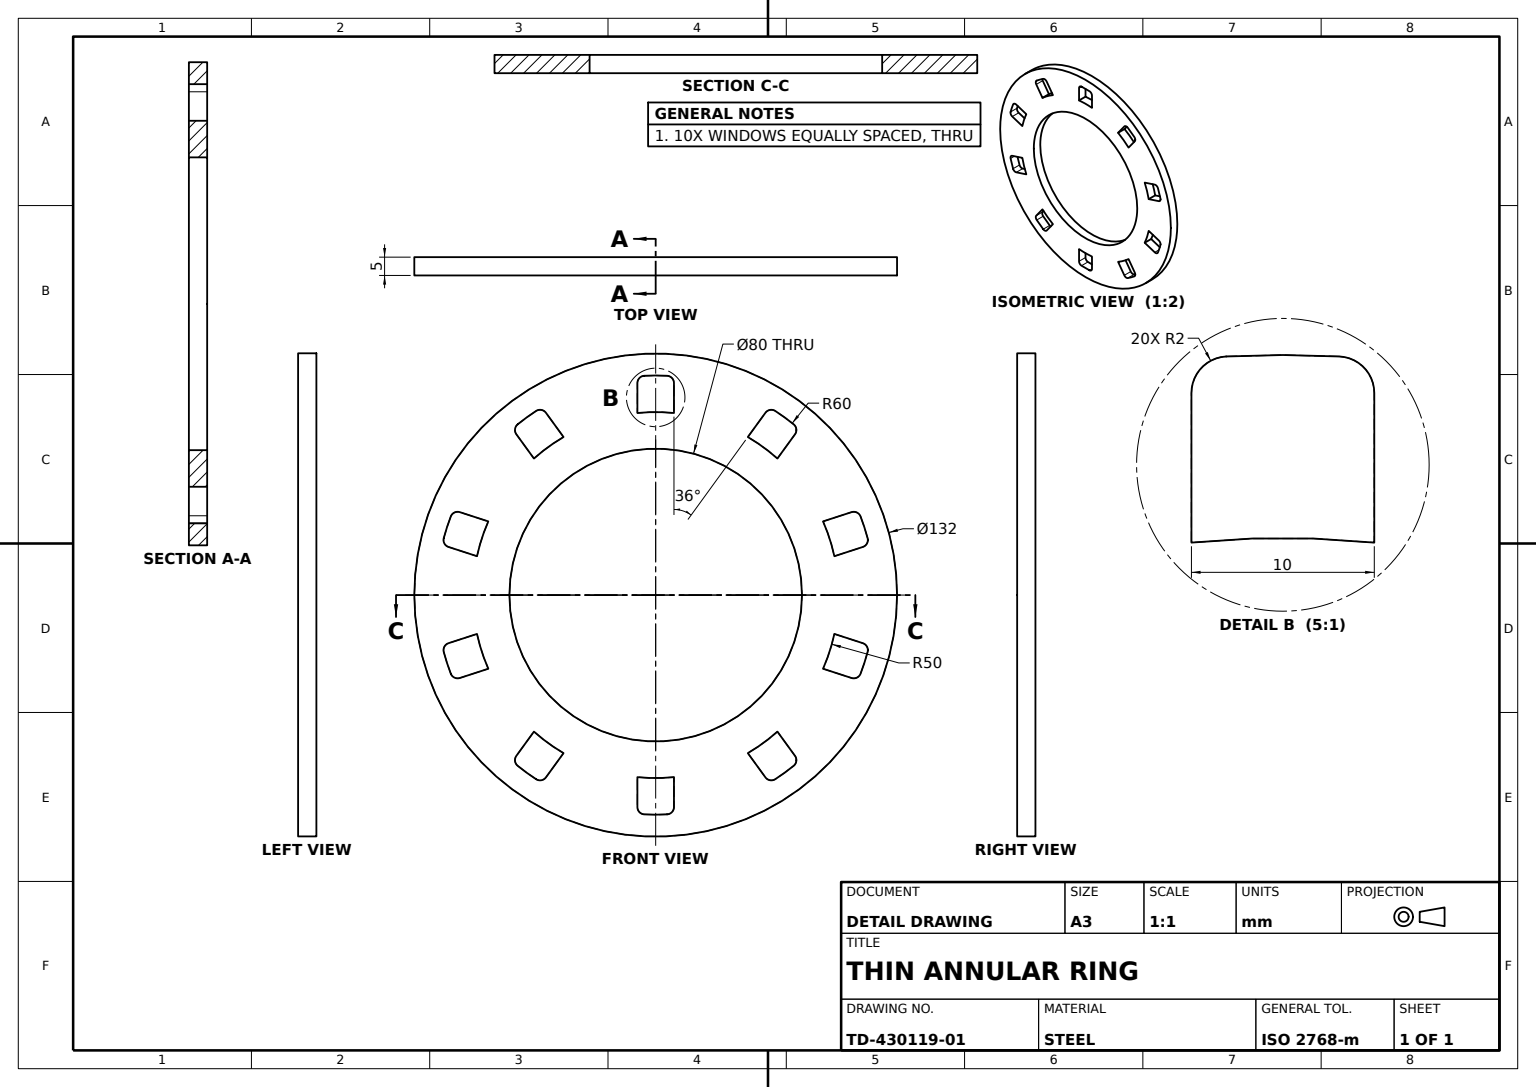
solid
v1 (-32.709165,50.300204,0)
v2 (-32.709165,50.300204,5)
e1 v1 v2 LINE
v3 (-37.730649,46.651882,5)
e2 v2 v3 CIRCLE(AX(P(0,0,5),D(0,0,1),D(0.809016994,0.587785252,0)),60)
v4 (-37.730649,46.651882,0)
e3 v4 v3 LINE
e4 v1 v4 CIRCLE(AX(P(0,0,0),D(0,0,1),D(1,0,0)),60)
face CYL(AX(P(0,0,-20),D(0,0,1),D(1,0,0)),60) rev [e1 e2 -e3 -e4]
v5 (-37.730649,-46.651882,5)
v6 (-32.709165,-50.300204,5)
e5 v5 v6 CIRCLE(AX(P(0,0,5),D(0,0,1),D(-0.809016994,0.587785252,0)),60)
v7 (-32.709165,-50.300204,0)
e6 v7 v6 LINE
v8 (-37.730649,-46.651882,0)
e7 v8 v7 CIRCLE(AX(P(0,0,0),D(0,0,1),D(1,0,0)),60)
e8 v8 v5 LINE
face CYL(AX(P(0,0,-20),D(0,0,1),D(1,0,0)),60) rev [e5 -e6 -e7 e8]
v9 (38.472961,-45.096819,5)
v10 (38.090995,-43.921249,5)
e9 v9 v10 CIRCLE(AX(P(36.472961,-45.096819,5),D(0,0,1),D(0.809016994,0.587785252,0)),2)
v11 (38.090995,-43.921249,0)
e10 v11 v10 LINE
v12 (38.472961,-45.096819,0)
e11 v12 v11 CIRCLE(AX(P(36.472961,-45.096819,0),D(0,0,1),D(1,0,0)),2)
e12 v12 v9 LINE
face CYL(AX(P(36.472961,-45.096819,-20),D(0,0,1),D(1,0,0)),2) rev [e9 -e10 -e11 e12]
v13 (57.946025,15.564646,0)
v14 (57.946025,15.564646,5)
e13 v13 v14 LINE
v15 (58.014491,15.045825,0)
e14 v15 v13 CIRCLE(AX(P(56.014491,15.045825,0),D(0,0,1),D(1,0,0)),2)
v16 (58.014491,15.045825,5)
e15 v15 v16 LINE
e16 v16 v14 CIRCLE(AX(P(56.014491,15.045825,5),D(0,0,1),D(0.309016994,-0.951056516,0)),2)
face CYL(AX(P(56.014491,15.045825,-20),D(0,0,1),D(1,0,0)),2) rev [-e13 -e14 e15 e16]
v17 (5,-49.749372,0)
v18 (-5,-49.749372,0)
e17 v17 v18 CIRCLE(AX(P(0,0,0),D(0,0,-1),D(1,0,0)),50)
v19 (5,-49.749372,5)
e18 v17 v19 LINE
v20 (-5,-49.749372,5)
e19 v19 v20 CIRCLE(AX(P(0,0,5),D(0,0,-1),D(-1,0,0)),50)
e20 v18 v20 LINE
face CYL(AX(P(0,0,-20),D(0,0,1),D(1,0,0)),50) [-e17 e18 e19 -e20]
v21 (53.542355,-22.654277,0)
v22 (53.542355,-22.654277,5)
e21 v21 v22 LINE
v23 (45.769379,-20.128684,0)
e22 v23 v21 LINE
v24 (45.769379,-20.128684,5)
e23 v23 v24 LINE
e24 v24 v22 LINE
face PLANE(AX(P(45.769379,-20.128684,-20),D(-0.309016994,-0.951056516,0),D(0.951056516,-0.309016994,0))) rev [-e21 -e22 e23 e24]
v25 (56.027988,21.467756,0)
v26 (56.027988,21.467756,5)
e25 v25 v26 LINE
e26 v13 v25 CIRCLE(AX(P(0,0,0),D(0,0,1),D(1,0,0)),60)
e27 v14 v26 CIRCLE(AX(P(0,0,5),D(0,0,1),D(0.309016994,-0.951056516,0)),60)
face CYL(AX(P(0,0,-20),D(0,0,1),D(1,0,0)),60) rev [-e25 -e26 e13 e27]
v27 (5,-57.922362,5)
e28 v27 v19 LINE
v28 (5,-57.922362,0)
e29 v28 v17 LINE
e30 v28 v27 LINE
face PLANE(AX(P(5,-57.922362,-20),D(1,0,0),D(0,1,0))) rev [e28 -e18 -e29 e30]
v29 (5,49.749372,5)
v30 (5,57.922362,5)
e31 v29 v30 LINE
v31 (5,57.922362,0)
e32 v31 v30 LINE
v32 (5,49.749372,0)
e33 v32 v31 LINE
e34 v32 v29 LINE
face PLANE(AX(P(5,49.749372,-20),D(1,0,0),D(0,1,0))) rev [e31 -e32 -e33 e34]
v33 (32.709165,50.300204,0)
v34 (32.709165,50.300204,5)
e35 v33 v34 LINE
v35 (30.000825,49.799101,5)
e36 v34 v35 CIRCLE(AX(P(31.618859,48.623531,5),D(0,0,1),D(-0.809016994,0.587785252,0)),2)
v36 (30.000825,49.799101,0)
e37 v36 v35 LINE
e38 v33 v36 CIRCLE(AX(P(31.618859,48.623531,0),D(0,0,1),D(1,0,0)),2)
face CYL(AX(P(31.618859,48.623531,-20),D(0,0,1),D(1,0,0)),2) rev [e35 e36 -e37 -e38]
v37 (-56.632525,-13.143712,0)
v38 (-57.946025,-15.564646,0)
e39 v37 v38 CIRCLE(AX(P(-56.014491,-15.045825,0),D(0,0,1),D(1,0,0)),2)
v39 (-56.632525,-13.143712,5)
e40 v37 v39 LINE
v40 (-57.946025,-15.564646,5)
e41 v39 v40 CIRCLE(AX(P(-56.014491,-15.045825,5),D(0,0,1),D(-0.309016994,0.951056516,0)),2)
e42 v38 v40 LINE
face CYL(AX(P(-56.014491,-15.045825,-20),D(0,0,1),D(1,0,0)),2) rev [-e39 e40 e41 -e42]
v41 (-40,0,5)
v42 (40,0,5)
e43 v41 v42 CIRCLE(AX(P(0,0,5),D(0,0,1),D(1,0,0)),40)
v43 (40,0,0)
e44 v43 v42 LINE
v44 (-40,0,0)
e45 v44 v43 CIRCLE(AX(P(0,0,0),D(0,0,1),D(1,0,0)),40)
e46 v44 v41 LINE
face CYL(AX(P(0,0,-20),D(0,0,1),D(1,0,0)),40) rev [e43 -e44 -e45 e46]
v45 (-56.027988,-21.467756,5)
e47 v40 v45 CIRCLE(AX(P(0,0,5),D(0,0,1),D(-0.309016994,0.951056516,0)),60)
v46 (-56.027988,-21.467756,0)
e48 v46 v45 LINE
e49 v38 v46 CIRCLE(AX(P(0,0,0),D(0,0,1),D(1,0,0)),60)
face CYL(AX(P(0,0,-20),D(0,0,1),D(1,0,0)),60) rev [e42 e47 -e48 -e49]
v47 (56.027988,-21.467756,0)
e50 v21 v47 CIRCLE(AX(P(54.160389,-20.752164,0),D(0,0,1),D(1,0,0)),2)
v48 (56.027988,-21.467756,5)
e51 v22 v48 CIRCLE(AX(P(54.160389,-20.752164,5),D(0,0,1),D(-0.309016994,-0.951056516,0)),2)
e52 v47 v48 LINE
face CYL(AX(P(54.160389,-20.752164,-20),D(0,0,1),D(1,0,0)),2) rev [-e50 e21 e51 -e52]
v49 (25.196862,43.187014,0)
v50 (33.287032,37.309161,0)
e53 v49 v50 CIRCLE(AX(P(0,0,0),D(0,0,-1),D(1,0,0)),50)
v51 (25.196862,43.187014,5)
e54 v49 v51 LINE
v52 (33.287032,37.309161,5)
e55 v51 v52 CIRCLE(AX(P(0,0,5),D(0,0,-1),D(0.809016994,-0.587785252,0)),50)
e56 v50 v52 LINE
face CYL(AX(P(0,0,-20),D(0,0,1),D(1,0,0)),50) [-e53 e54 e55 -e56]
v53 (-45.769379,-20.128684,0)
v54 (-45.769379,-20.128684,5)
e57 v53 v54 LINE
v55 (-48.859549,-10.618119,5)
e58 v54 v55 CIRCLE(AX(P(0,0,5),D(0,0,-1),D(-0.309016994,0.951056516,0)),50)
v56 (-48.859549,-10.618119,0)
e59 v56 v55 LINE
e60 v53 v56 CIRCLE(AX(P(0,0,0),D(0,0,-1),D(1,0,0)),50)
face CYL(AX(P(0,0,-20),D(0,0,1),D(1,0,0)),50) [e57 e58 -e59 -e60]
v57 (-33.287032,-37.309161,0)
v58 (-33.287032,-37.309161,5)
e61 v57 v58 LINE
v59 (-38.090995,-43.921249,5)
e62 v58 v59 LINE
v60 (-38.090995,-43.921249,0)
e63 v60 v59 LINE
e64 v57 v60 LINE
face PLANE(AX(P(-33.287032,-37.309161,-20),D(-0.809016994,0.587785252,0),D(-0.587785252,-0.809016994,0))) rev [e61 e62 -e63 -e64]
v61 (-30.000825,49.799101,5)
e65 v61 v2 CIRCLE(AX(P(-31.618859,48.623531,5),D(0,0,1),D(0.809016994,0.587785252,0)),2)
v62 (-25.196862,43.187014,5)
e66 v62 v61 LINE
v63 (-33.287032,37.309161,5)
e67 v63 v62 CIRCLE(AX(P(0,0,5),D(0,0,-1),D(0.809016994,0.587785252,0)),50)
v64 (-38.090995,43.921249,5)
e68 v64 v63 LINE
e69 v3 v64 CIRCLE(AX(P(-36.472961,45.096819,5),D(0,0,1),D(-0.809016994,-0.587785252,0)),2)
v65 (-25.196862,-43.187014,5)
e70 v65 v58 CIRCLE(AX(P(0,0,5),D(0,0,-1),D(-0.809016994,0.587785252,0)),50)
v66 (-30.000825,-49.799101,5)
e71 v66 v65 LINE
e72 v6 v66 CIRCLE(AX(P(-31.618859,-48.623531,5),D(0,0,1),D(0.809016994,-0.587785252,0)),2)
e73 v59 v5 CIRCLE(AX(P(-36.472961,-45.096819,5),D(0,0,1),D(-0.809016994,0.587785252,0)),2)
v67 (56.632525,13.143712,5)
e74 v67 v16 CIRCLE(AX(P(56.014491,15.045825,5),D(0,0,1),D(0.309016994,-0.951056516,0)),2)
v68 (48.859549,10.618119,5)
e75 v68 v67 LINE
v69 (45.769379,20.128684,5)
e76 v69 v68 CIRCLE(AX(P(0,0,5),D(0,0,-1),D(0.309016994,-0.951056516,0)),50)
v70 (53.542355,22.654277,5)
e77 v70 v69 LINE
e78 v26 v70 CIRCLE(AX(P(54.160389,20.752164,5),D(0,0,1),D(-0.309016994,0.951056516,0)),2)
v71 (-57.946025,15.564646,5)
v72 (-56.632525,13.143712,5)
e79 v71 v72 CIRCLE(AX(P(-56.014491,15.045825,5),D(0,0,1),D(-0.309016994,-0.951056516,0)),2)
v73 (-56.027988,21.467756,5)
e80 v73 v71 CIRCLE(AX(P(0,0,5),D(0,0,1),D(0.309016994,0.951056516,0)),60)
v74 (-53.542355,22.654277,5)
e81 v74 v73 CIRCLE(AX(P(-54.160389,20.752164,5),D(0,0,1),D(0.309016994,0.951056516,0)),2)
v75 (-45.769379,20.128684,5)
e82 v75 v74 LINE
v76 (-48.859549,10.618119,5)
e83 v76 v75 CIRCLE(AX(P(0,0,5),D(0,0,-1),D(0.309016994,0.951056516,0)),50)
e84 v72 v76 LINE
e85 v35 v51 LINE
v77 (37.730649,46.651882,5)
e86 v77 v34 CIRCLE(AX(P(0,0,5),D(0,0,1),D(0.809016994,-0.587785252,0)),60)
v78 (38.472961,45.096819,5)
e87 v78 v77 CIRCLE(AX(P(36.472961,45.096819,5),D(0,0,1),D(0.809016994,-0.587785252,0)),2)
v79 (38.090995,43.921249,5)
e88 v79 v78 CIRCLE(AX(P(36.472961,45.096819,5),D(0,0,1),D(0.809016994,-0.587785252,0)),2)
e89 v52 v79 LINE
v80 (66,0,5)
v81 (-66,0,5)
e90 v80 v81 CIRCLE(AX(P(0,0,5),D(0,0,1),D(1,0,0)),66)
e91 v81 v80 CIRCLE(AX(P(0,0,5),D(0,0,1),D(1,0,0)),66)
e92 v55 v39 LINE
v82 (-53.542355,-22.654277,5)
e93 v82 v54 LINE
e94 v45 v82 CIRCLE(AX(P(-54.160389,-20.752164,5),D(0,0,1),D(0.309016994,-0.951056516,0)),2)
v83 (32.709165,-50.300204,5)
v84 (37.730649,-46.651882,5)
e95 v83 v84 CIRCLE(AX(P(0,0,5),D(0,0,1),D(-0.809016994,-0.587785252,0)),60)
v85 (30.000825,-49.799101,5)
e96 v85 v83 CIRCLE(AX(P(31.618859,-48.623531,5),D(0,0,1),D(-0.809016994,-0.587785252,0)),2)
v86 (25.196862,-43.187014,5)
e97 v86 v85 LINE
v87 (33.287032,-37.309161,5)
e98 v87 v86 CIRCLE(AX(P(0,0,5),D(0,0,-1),D(-0.809016994,-0.587785252,0)),50)
e99 v10 v87 LINE
e100 v84 v9 CIRCLE(AX(P(36.472961,-45.096819,5),D(0,0,1),D(0.809016994,0.587785252,0)),2)
e101 v42 v41 CIRCLE(AX(P(0,0,5),D(0,0,1),D(1,0,0)),40)
v88 (3.103448,59.919685,5)
v89 (-3.103448,59.919685,5)
e102 v88 v89 CIRCLE(AX(P(0,0,5),D(0,0,1),D(1,0,0)),60)
e103 v30 v88 CIRCLE(AX(P(3,57.922362,5),D(0,0,1),D(1,0,0)),2)
v90 (-5,49.749372,5)
e104 v90 v29 CIRCLE(AX(P(0,0,5),D(0,0,-1),D(1,0,0)),50)
v91 (-5,57.922362,5)
e105 v91 v90 LINE
e106 v89 v91 CIRCLE(AX(P(-3,57.922362,5),D(0,0,1),D(-1,0,0)),2)
v92 (-5,-57.922362,5)
e107 v20 v92 LINE
v93 (3.103448,-59.919685,5)
e108 v93 v27 CIRCLE(AX(P(3,-57.922362,5),D(0,0,1),D(1,0,0)),2)
v94 (-3.103448,-59.919685,5)
e109 v94 v93 CIRCLE(AX(P(0,0,5),D(0,0,1),D(-1,0,0)),60)
e110 v92 v94 CIRCLE(AX(P(-3,-57.922362,5),D(0,0,1),D(-1,0,0)),2)
v95 (57.946025,-15.564646,5)
e111 v48 v95 CIRCLE(AX(P(0,0,5),D(0,0,1),D(-0.309016994,-0.951056516,0)),60)
v96 (48.859549,-10.618119,5)
e112 v96 v24 CIRCLE(AX(P(0,0,5),D(0,0,-1),D(-0.309016994,-0.951056516,0)),50)
v97 (56.632525,-13.143712,5)
e113 v97 v96 LINE
v98 (58.014491,-15.045825,5)
e114 v98 v97 CIRCLE(AX(P(56.014491,-15.045825,5),D(0,0,1),D(0.309016994,0.951056516,0)),2)
e115 v95 v98 CIRCLE(AX(P(56.014491,-15.045825,5),D(0,0,1),D(0.309016994,0.951056516,0)),2)
face PLANE(AX(P(0,0,5),D(0,0,1),D(1,0,0))) [-e65 -e66 -e67 -e68 -e69 -e2] [-e70 -e71 -e72 -e5 -e73 -e62] [-e27 -e16 -e74 -e75 -e76 -e77 -e78] [-e79 -e80 -e81 -e82 -e83 -e84] [-e55 -e85 -e36 -e86 -e87 -e88 -e89] [e90 e91] [-e47 -e41 -e92 -e58 -e93 -e94] [-e95 -e96 -e97 -e98 -e99 -e9 -e100] [-e43 -e101] [-e102 -e103 -e31 -e104 -e105 -e106] [-e107 -e19 -e28 -e108 -e109 -e110] [-e111 -e51 -e24 -e112 -e113 -e114 -e115]
v99 (33.287032,-37.309161,0)
e116 v99 v87 LINE
e117 v11 v99 LINE
face PLANE(AX(P(38.090995,-43.921249,-20),D(0.809016994,0.587785252,0),D(-0.587785252,0.809016994,0))) rev [-e116 -e117 e10 e99]
v100 (-38.090995,43.921249,0)
e118 v100 v64 LINE
v101 (-33.287032,37.309161,0)
e119 v101 v63 LINE
e120 v100 v101 LINE
face PLANE(AX(P(-38.090995,43.921249,-20),D(-0.809016994,-0.587785252,0),D(0.587785252,-0.809016994,0))) rev [e118 e68 -e119 -e120]
v102 (30.000825,-49.799101,0)
e121 v102 v85 LINE
v103 (25.196862,-43.187014,0)
e122 v103 v102 LINE
e123 v103 v86 LINE
face PLANE(AX(P(25.196862,-43.187014,-20),D(-0.809016994,-0.587785252,0),D(0.587785252,-0.809016994,0))) rev [-e121 -e122 e123 e97]
v104 (38.472961,45.096819,0)
e124 v104 v78 LINE
v105 (37.730649,46.651882,0)
e125 v105 v77 LINE
e126 v104 v105 CIRCLE(AX(P(36.472961,45.096819,0),D(0,0,1),D(1,0,0)),2)
face CYL(AX(P(36.472961,45.096819,-20),D(0,0,1),D(1,0,0)),2) rev [e124 e87 -e125 -e126]
e127 v99 v103 CIRCLE(AX(P(0,0,0),D(0,0,-1),D(1,0,0)),50)
face CYL(AX(P(0,0,-20),D(0,0,1),D(1,0,0)),50) [e116 e98 -e123 -e127]
v106 (38.090995,43.921249,0)
e128 v106 v79 LINE
e129 v50 v106 LINE
face PLANE(AX(P(33.287032,37.309161,-20),D(0.809016994,-0.587785252,0),D(0.587785252,0.809016994,0))) rev [e56 e89 -e128 -e129]
v107 (-53.542355,22.654277,0)
e130 v107 v74 LINE
v108 (-45.769379,20.128684,0)
e131 v108 v107 LINE
e132 v108 v75 LINE
face PLANE(AX(P(-45.769379,20.128684,-20),D(0.309016994,0.951056516,0),D(-0.951056516,0.309016994,0))) rev [e82 -e130 -e131 e132]
v109 (-5,-57.922362,0)
e133 v109 v92 LINE
e134 v18 v109 LINE
face PLANE(AX(P(-5,-49.749372,-20),D(-1,0,0),D(0,-1,0))) rev [e107 -e133 -e134 e20]
e135 v106 v104 CIRCLE(AX(P(36.472961,45.096819,0),D(0,0,1),D(1,0,0)),2)
face CYL(AX(P(36.472961,45.096819,-20),D(0,0,1),D(1,0,0)),2) rev [-e124 -e135 e128 e88]
v110 (-66,0,0)
v111 (66,0,0)
e136 v110 v111 CIRCLE(AX(P(0,0,0),D(0,0,1),D(1,0,0)),66)
e137 v80 v111 LINE
e138 v81 v110 LINE
face CYL(AX(P(0,0,5),D(0,0,-1),D(-1,0,0)),66) [e136 -e137 -e91 e138]
v112 (-48.859549,10.618119,0)
e139 v112 v76 LINE
v113 (-56.632525,13.143712,0)
e140 v113 v112 LINE
e141 v113 v72 LINE
face PLANE(AX(P(-56.632525,13.143712,-20),D(-0.309016994,-0.951056516,0),D(0.951056516,-0.309016994,0))) rev [e84 -e139 -e140 e141]
v114 (-56.027988,21.467756,0)
e142 v107 v114 CIRCLE(AX(P(-54.160389,20.752164,0),D(0,0,1),D(1,0,0)),2)
e143 v114 v73 LINE
face CYL(AX(P(-54.160389,20.752164,-20),D(0,0,1),D(1,0,0)),2) rev [-e142 e130 e81 -e143]
v115 (-30.000825,-49.799101,0)
e144 v7 v115 CIRCLE(AX(P(-31.618859,-48.623531,0),D(0,0,1),D(1,0,0)),2)
e145 v115 v66 LINE
face CYL(AX(P(-31.618859,-48.623531,-20),D(0,0,1),D(1,0,0)),2) rev [-e144 e6 e72 -e145]
e146 v111 v110 CIRCLE(AX(P(0,0,0),D(0,0,1),D(1,0,0)),66)
face CYL(AX(P(0,0,5),D(0,0,-1),D(-1,0,0)),66) [e146 -e138 -e90 e137]
e147 v36 v49 LINE
face PLANE(AX(P(30.000825,49.799101,-20),D(-0.809016994,0.587785252,0),D(-0.587785252,-0.809016994,0))) rev [-e54 -e147 e37 e85]
v116 (58.014491,-15.045825,0)
e148 v116 v98 LINE
v117 (56.632525,-13.143712,0)
e149 v117 v97 LINE
e150 v116 v117 CIRCLE(AX(P(56.014491,-15.045825,0),D(0,0,1),D(1,0,0)),2)
face CYL(AX(P(56.014491,-15.045825,-20),D(0,0,1),D(1,0,0)),2) rev [e148 e114 -e149 -e150]
v118 (3.103448,59.919685,0)
e151 v118 v88 LINE
e152 v31 v118 CIRCLE(AX(P(3,57.922362,0),D(0,0,1),D(1,0,0)),2)
face CYL(AX(P(3,57.922362,-20),D(0,0,1),D(1,0,0)),2) rev [e32 e103 -e151 -e152]
v119 (-57.946025,15.564646,0)
e153 v119 v113 CIRCLE(AX(P(-56.014491,15.045825,0),D(0,0,1),D(1,0,0)),2)
e154 v119 v71 LINE
face CYL(AX(P(-56.014491,15.045825,-20),D(0,0,1),D(1,0,0)),2) rev [-e141 -e153 e154 e79]
v120 (57.946025,-15.564646,0)
e155 v120 v95 LINE
e156 v47 v120 CIRCLE(AX(P(0,0,0),D(0,0,1),D(1,0,0)),60)
face CYL(AX(P(0,0,-20),D(0,0,1),D(1,0,0)),60) rev [e52 e111 -e155 -e156]
v121 (32.709165,-50.300204,0)
e157 v102 v121 CIRCLE(AX(P(31.618859,-48.623531,0),D(0,0,1),D(1,0,0)),2)
e158 v121 v83 LINE
face CYL(AX(P(31.618859,-48.623531,-20),D(0,0,1),D(1,0,0)),2) rev [-e157 e121 e96 -e158]
v122 (56.632525,13.143712,0)
e159 v122 v15 CIRCLE(AX(P(56.014491,15.045825,0),D(0,0,1),D(1,0,0)),2)
e160 v122 v67 LINE
face CYL(AX(P(56.014491,15.045825,-20),D(0,0,1),D(1,0,0)),2) rev [-e159 e160 e74 -e15]
v123 (37.730649,-46.651882,0)
e161 v123 v84 LINE
e162 v121 v123 CIRCLE(AX(P(0,0,0),D(0,0,1),D(1,0,0)),60)
face CYL(AX(P(0,0,-20),D(0,0,1),D(1,0,0)),60) rev [-e161 -e162 e158 e95]
v124 (3.103448,-59.919685,0)
e163 v124 v28 CIRCLE(AX(P(3,-57.922362,0),D(0,0,1),D(1,0,0)),2)
e164 v124 v93 LINE
face CYL(AX(P(3,-57.922362,-20),D(0,0,1),D(1,0,0)),2) rev [e108 -e30 -e163 e164]
v125 (48.859549,-10.618119,0)
e165 v125 v96 LINE
e166 v125 v23 CIRCLE(AX(P(0,0,0),D(0,0,-1),D(1,0,0)),50)
face CYL(AX(P(0,0,-20),D(0,0,1),D(1,0,0)),50) [e165 e112 -e23 -e166]
v126 (-30.000825,49.799101,0)
e167 v126 v1 CIRCLE(AX(P(-31.618859,48.623531,0),D(0,0,1),D(1,0,0)),2)
e168 v126 v61 LINE
face CYL(AX(P(-31.618859,48.623531,-20),D(0,0,1),D(1,0,0)),2) rev [e65 -e1 -e167 e168]
e169 v56 v37 LINE
face PLANE(AX(P(-48.859549,-10.618119,-20),D(-0.309016994,0.951056516,0),D(-0.951056516,-0.309016994,0))) rev [-e169 e59 e92 -e40]
e170 v114 v119 CIRCLE(AX(P(0,0,0),D(0,0,1),D(1,0,0)),60)
face CYL(AX(P(0,0,-20),D(0,0,1),D(1,0,0)),60) rev [-e154 -e170 e143 e80]
v127 (-53.542355,-22.654277,0)
e171 v127 v82 LINE
e172 v46 v127 CIRCLE(AX(P(-54.160389,-20.752164,0),D(0,0,1),D(1,0,0)),2)
face CYL(AX(P(-54.160389,-20.752164,-20),D(0,0,1),D(1,0,0)),2) rev [e94 -e171 -e172 e48]
v128 (-25.196862,43.187014,0)
e173 v128 v62 LINE
e174 v128 v126 LINE
face PLANE(AX(P(-25.196862,43.187014,-20),D(0.809016994,0.587785252,0),D(-0.587785252,0.809016994,0))) rev [e173 e66 -e168 -e174]
v129 (-3.103448,59.919685,0)
e175 v129 v89 LINE
e176 v118 v129 CIRCLE(AX(P(0,0,0),D(0,0,1),D(1,0,0)),60)
face CYL(AX(P(0,0,-20),D(0,0,1),D(1,0,0)),60) rev [-e175 -e176 e151 e102]
e177 v120 v116 CIRCLE(AX(P(56.014491,-15.045825,0),D(0,0,1),D(1,0,0)),2)
face CYL(AX(P(56.014491,-15.045825,-20),D(0,0,1),D(1,0,0)),2) rev [-e148 -e177 e155 e115]
e178 v112 v108 CIRCLE(AX(P(0,0,0),D(0,0,-1),D(1,0,0)),50)
face CYL(AX(P(0,0,-20),D(0,0,1),D(1,0,0)),50) [e83 -e132 -e178 e139]
v130 (48.859549,10.618119,0)
e179 v130 v68 LINE
e180 v130 v122 LINE
face PLANE(AX(P(48.859549,10.618119,-20),D(0.309016994,-0.951056516,0),D(0.951056516,0.309016994,0))) rev [e179 e75 -e160 -e180]
e181 v4 v100 CIRCLE(AX(P(-36.472961,45.096819,0),D(0,0,1),D(1,0,0)),2)
face CYL(AX(P(-36.472961,45.096819,-20),D(0,0,1),D(1,0,0)),2) rev [e3 e69 -e118 -e181]
v131 (-25.196862,-43.187014,0)
e182 v131 v57 CIRCLE(AX(P(0,0,0),D(0,0,-1),D(1,0,0)),50)
e183 v131 v65 LINE
face CYL(AX(P(0,0,-20),D(0,0,1),D(1,0,0)),50) [-e61 -e182 e183 e70]
e184 v117 v125 LINE
face PLANE(AX(P(56.632525,-13.143712,-20),D(0.309016994,0.951056516,0),D(-0.951056516,0.309016994,0))) rev [-e184 e149 e113 -e165]
v132 (45.769379,20.128684,0)
e185 v132 v69 LINE
v133 (53.542355,22.654277,0)
e186 v133 v132 LINE
e187 v133 v70 LINE
face PLANE(AX(P(53.542355,22.654277,-20),D(-0.309016994,0.951056516,0),D(-0.951056516,-0.309016994,0))) rev [e77 -e185 -e186 e187]
v134 (-3.103448,-59.919685,0)
e188 v109 v134 CIRCLE(AX(P(-3,-57.922362,0),D(0,0,1),D(1,0,0)),2)
e189 v134 v94 LINE
face CYL(AX(P(-3,-57.922362,-20),D(0,0,1),D(1,0,0)),2) rev [-e188 e133 e110 -e189]
e190 v60 v8 CIRCLE(AX(P(-36.472961,-45.096819,0),D(0,0,1),D(1,0,0)),2)
face CYL(AX(P(-36.472961,-45.096819,-20),D(0,0,1),D(1,0,0)),2) rev [-e8 -e190 e63 e73]
e191 v105 v33 CIRCLE(AX(P(0,0,0),D(0,0,1),D(1,0,0)),60)
face CYL(AX(P(0,0,-20),D(0,0,1),D(1,0,0)),60) rev [e125 e86 -e35 -e191]
e192 v115 v131 LINE
face PLANE(AX(P(-30.000825,-49.799101,-20),D(0.809016994,-0.587785252,0),D(0.587785252,0.809016994,0))) rev [e145 e71 -e183 -e192]
e193 v101 v128 CIRCLE(AX(P(0,0,0),D(0,0,-1),D(1,0,0)),50)
face CYL(AX(P(0,0,-20),D(0,0,1),D(1,0,0)),50) [-e173 -e193 e119 e67]
e194 v25 v133 CIRCLE(AX(P(54.160389,20.752164,0),D(0,0,1),D(1,0,0)),2)
face CYL(AX(P(54.160389,20.752164,-20),D(0,0,1),D(1,0,0)),2) rev [-e194 e25 e78 -e187]
v135 (-5,49.749372,0)
e195 v135 v90 LINE
e196 v135 v32 CIRCLE(AX(P(0,0,0),D(0,0,-1),D(1,0,0)),50)
face CYL(AX(P(0,0,-20),D(0,0,1),D(1,0,0)),50) [e195 e104 -e34 -e196]
e197 v127 v53 LINE
e198 v43 v44 CIRCLE(AX(P(0,0,0),D(0,0,1),D(1,0,0)),40)
e199 v134 v124 CIRCLE(AX(P(0,0,0),D(0,0,1),D(1,0,0)),60)
e200 v132 v130 CIRCLE(AX(P(0,0,0),D(0,0,-1),D(1,0,0)),50)
e201 v123 v12 CIRCLE(AX(P(36.472961,-45.096819,0),D(0,0,1),D(1,0,0)),2)
v136 (-5,57.922362,0)
e202 v129 v136 CIRCLE(AX(P(-3,57.922362,0),D(0,0,1),D(1,0,0)),2)
e203 v136 v135 LINE
face PLANE(AX(P(0,0,0),D(0,0,1),D(1,0,0))) rev [e170 e153 e140 e178 e131 e142] [e191 e38 e147 e53 e129 e135 e126] [e60 e169 e39 e49 e172 e197] [-e136 -e146] [e45 e198] [e199 e163 e29 e17 e134 e188] [e22 e50 e156 e177 e150 e184 e166] [e167 e4 e181 e120 e193 e174] [e194 e186 e200 e180 e159 e14 e26] [e127 e122 e157 e162 e201 e11 e117] [e192 e182 e64 e190 e7 e144] [e176 e202 e203 e196 e33 e152]
face CYL(AX(P(36.472961,-45.096819,-20),D(0,0,1),D(1,0,0)),2) rev [e100 -e12 -e201 e161]
e204 v136 v91 LINE
face PLANE(AX(P(-5,57.922362,-20),D(-1,0,0),D(0,-1,0))) rev [e105 -e195 -e203 e204]
face CYL(AX(P(0,0,-20),D(0,0,1),D(1,0,0)),60) rev [e109 -e164 -e199 e189]
face PLANE(AX(P(-53.542355,-22.654277,-20),D(0.309016994,-0.951056516,0),D(0.951056516,0.309016994,0))) rev [-e57 -e197 e171 e93]
face CYL(AX(P(0,0,-20),D(0,0,1),D(1,0,0)),50) [-e179 -e200 e185 e76]
face CYL(AX(P(-3,57.922362,-20),D(0,0,1),D(1,0,0)),2) rev [-e204 -e202 e175 e106]
face CYL(AX(P(0,0,-20),D(0,0,1),D(1,0,0)),40) rev [-e198 e44 e101 -e46]
